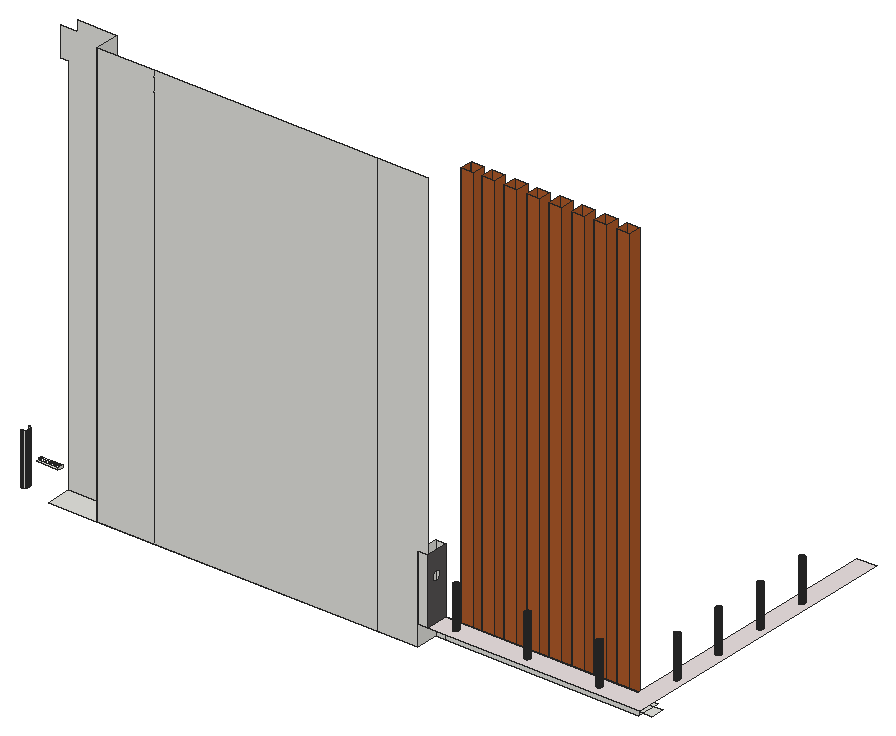
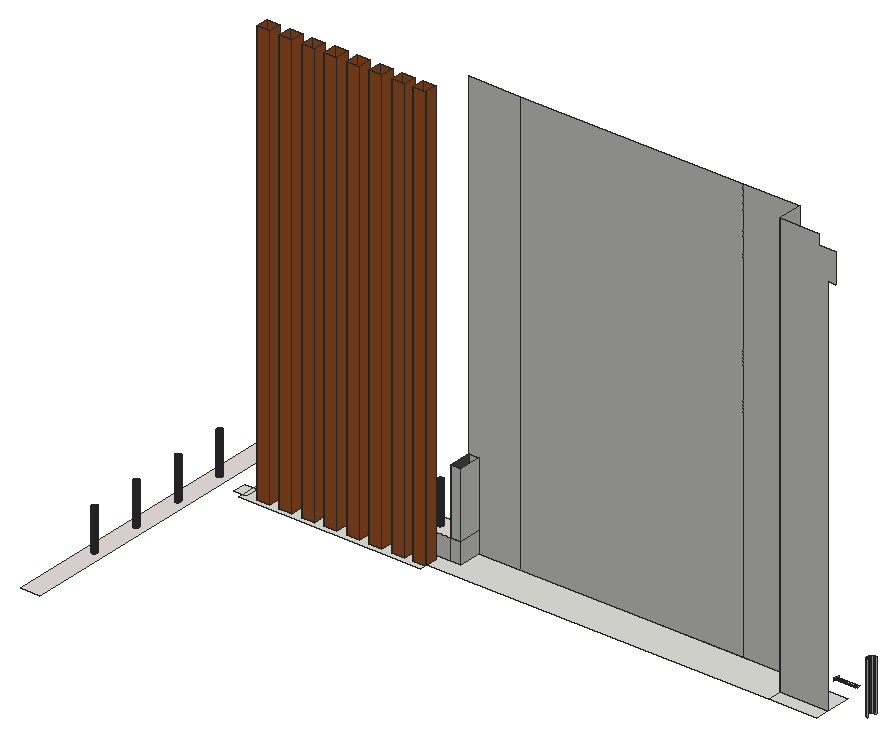
# SketchUp Ruby script. Lengths in inches.
U = 1.inch
M = Sketchup.active_model
def pt(a) = Geom::Point3d.new(a.map { |v| v * U })
def face(e, loops, mat)
  f = e.add_face(loops[0].map { |a| pt(a) })
  loops[1..].each { |l| e.add_face(l.map { |a| pt(a) }).erase! }
  f.material = f.back_material = mat if mat
  f
end
# faces: each face lists its corners as indices into pts; further lists are holes
def faces(e, pts, list, mat = nil) = list.each { |f| face(e, (f[0].is_a?(Array) ? f : [f]).map { |l| l.map { |i| pts[i] } }, mat) }
# xy, xz, yz: faces in a plane at the given z, y or x. An outline is a flat list of corners, or four numbers for a rectangle; further outlines are holes
def ring(l) = l.size == 4 ? [[l[0], l[1]], [l[2], l[1]], [l[2], l[3]], [l[0], l[3]]] : l.each_slice(2).to_a
def flat(e, list, mat, &to3) = list.each { |f| face(e, (f[0].is_a?(Array) ? f : [f]).map { |l| ring(l).map { |u, v| to3.(u, v) } }, mat) }
def xy(e, z, list, mat = nil) = flat(e, list, mat) { |x, y| [x, y, z] }
def xz(e, y, list, mat = nil) = flat(e, list, mat) { |x, z| [x, y, z] }
def yz(e, x, list, mat = nil) = flat(e, list, mat) { |y, z| [x, y, z] }
def lines(e, pts, list) = list.each { |a, b| e.add_line(pt(pts[a]), pt(pts[b])) }
# prism: a flat outline (further loops are holes) pulled along v
def prism(e, loops, v, mat = nil)
  f = face(e, loops, mat); d = Geom::Vector3d.new(v.map { |x| x * U })
  f.pushpull(f.normal.samedirection?(d) ? d.length : -d.length)
end
def box(e, o, s, mat = nil) = prism(e, [[o, [o[0] + s[0], o[1], o[2]], [o[0] + s[0], o[1] + s[1], o[2]], [o[0], o[1] + s[1], o[2]]]], [0, 0, s[2]], mat)
def at(x, y, z, deg = 0) = Geom::Transformation.translation(pt([x, y, z])) * Geom::Transformation.rotation(ORIGIN, Z_AXIS, deg.degrees)
def axes(o, x, y, z) = Geom::Transformation.new([*x, 0, *y, 0, *z, 0, *pt(o).to_a, 1])
def part(name) = M.definitions.add(name)
# library, detail: a bought-in or finely detailed component or shape, given as its bounding box
def library(name, o, s) = part(name).tap { |d| box(d.entities, o, s) }
def detail(e, o, s) = box(e.add_group.entities, o, s)
def put(e, d, t, mat = nil) = e.add_instance(d, t).tap { |i| i.material = mat if mat }
def group(e, t, mat = nil) = e.add_group.tap { |g| g.transformation = t; g.material = mat if mat }.entities
root = M.entities
M.materials.add("Generic\#2").color = [87, 84, 84]
M.materials.add("Generic\#6").color = [174, 89, 41]
M.materials.add("Generic\#9").color = [233, 223, 223]
M.materials.add("[Color M07]").color = [58, 58, 58]
xy(root,143.28,[[383.85,127.4375,394.85,133.125],[[394.85,127.4375,467.91,127.4375,467.91,132.5625,514.25,132.5625,514.25,133.85,513.34,133.85,513.34,136.78,514.25,136.78,514.25,138,472.76,138,472.76,136.78,475.69,136.78,475.69,133.85,472.76,133.85,472.76,136.1875,394.85,136.1875],[508.21,133.85,511.15,136.78],[503.09,133.85,506.03,136.78],[497.96,133.85,500.9,136.78],[492.84,133.85,495.78,136.78],[487.71,133.85,490.65,136.78],[482.59,133.85,485.53,136.78],[477.46,133.85,480.4,136.78]],[383.85,133.125,394.85,136.1875],[513.34,133.85,514.25,136.78],[514.25,133.85,516.28,136.78]])
xy(root,148.0625,[[467.91,127.4375,470.29,132.5625]])
xy(root,148.0625,[[[470.29,127.4375,518.6875,127.4375,518.6875,194.75,514.25,194.75,514.25,132.5625,470.29,132.5625],[516.54,175.625,516.38,175.65,516.23,175.71,516.1,175.81,516,175.9375,515.9375,176.09,515.92,176.25,515.9375,176.41,516,176.5625,516.1,176.69,516.23,176.79,516.38,176.85,516.54,176.875,516.7,176.85,516.86,176.79,516.98,176.69,517.08,176.5625,517.15,176.41,517.17,176.25,517.15,176.09,517.08,175.9375,516.98,175.81,516.86,175.71,516.7,175.65],[516.54,140,516.38,140.02,516.23,140.08,516.1,140.18,516,140.3125,515.9375,140.46,515.92,140.625,515.9375,140.79,516,140.9375,516.1,141.07,516.23,141.17,516.38,141.23,516.54,141.25,516.7,141.23,516.86,141.17,516.98,141.07,517.08,140.9375,517.15,140.79,517.17,140.625,517.15,140.46,517.08,140.3125,516.98,140.18,516.86,140.08,516.7,140.02],[516.54,151.875,516.38,151.9,516.23,151.96,516.1,152.06,516,152.1875,515.9375,152.34,515.92,152.5,515.9375,152.66,516,152.8125,516.1,152.94,516.23,153.04,516.38,153.1,516.54,153.125,516.7,153.1,516.86,153.04,516.98,152.94,517.08,152.8125,517.15,152.66,517.17,152.5,517.15,152.34,517.08,152.1875,516.98,152.06,516.86,151.96,516.7,151.9],[516.54,163.75,516.38,163.77,516.23,163.83,516.1,163.93,516,164.0625,515.9375,164.21,515.92,164.375,515.9375,164.54,516,164.6875,516.1,164.82,516.23,164.92,516.38,164.98,516.54,165,516.7,164.98,516.86,164.92,516.98,164.82,517.08,164.6875,517.15,164.54,517.17,164.375,517.15,164.21,517.08,164.0625,516.98,163.93,516.86,163.83,516.7,163.77],[490.99,129.43,490.83,129.45,490.68,129.51,490.55,129.61,490.45,129.74,490.39,129.89,490.37,130.05,490.39,130.21,490.45,130.36,490.55,130.49,490.68,130.59,490.83,130.66,490.99,130.68,491.15,130.66,491.3,130.59,491.43,130.49,491.53,130.36,491.59,130.21,491.62,130.05,491.59,129.89,491.53,129.74,491.43,129.61,491.3,129.51,491.15,129.45],[507.37,129.43,507.2,129.45,507.05,129.51,506.92,129.61,506.82,129.74,506.76,129.89,506.74,130.05,506.76,130.21,506.82,130.36,506.92,130.49,507.05,130.59,507.2,130.66,507.37,130.68,507.53,130.66,507.68,130.59,507.81,130.49,507.91,130.36,507.97,130.21,507.99,130.05,507.97,129.89,507.91,129.74,507.81,129.61,507.68,129.51,507.53,129.45],[474.62,129.43,474.45,129.45,474.3,129.51,474.17,129.61,474.07,129.74,474.01,129.89,473.99,130.05,474.01,130.21,474.07,130.36,474.17,130.49,474.3,130.59,474.45,130.66,474.62,130.68,474.78,130.66,474.93,130.59,475.06,130.49,475.16,130.36,475.22,130.21,475.24,130.05,475.22,129.89,475.16,129.74,475.06,129.61,474.93,129.51,474.78,129.45]]],"Generic\#9")
xy(root,148.75,[[378.85,130.19,383.85,130.82]])
xz(root,127.4375,[[394.85,143.28,407.84,240],[407.84,143.28,458.64,240],[458.64,143.28,458.64,240,470.29,240,470.29,162.875,467.91,162.875,467.91,143.28],[467.91,148.0625,470.29,162.875]])
xz(root,130.82,[[378.85,149.0625,383.85,149.1875],[378.85,149.0625,383.85,149.1875]])
xz(root,132.5625,[[467.91,143.28,470.29,148.0625],[470.29,143.28,514.25,148.0625],[467.91,148.0625,470.29,162.875]])
xz(root,133.125,[[383.85,143.28,383.85,231,381.97,231,381.97,237.6875,385.91,237.6875,385.91,240,394.85,240,394.85,143.28]])
xz(root,133.85,[[472.76,143.28,475.69,240],[477.46,143.28,480.4,240],[482.59,143.28,485.53,240],[487.71,143.28,490.65,240],[492.84,143.28,495.78,240],
  [497.96,143.28,500.9,240],[503.09,143.28,506.03,240],[508.21,143.28,511.15,240]],"Generic\#6")
xz(root,136.78,[[472.76,143.28,475.69,240],[477.46,143.28,480.4,240],[482.59,143.28,485.53,240],[487.71,143.28,490.65,240],[492.84,143.28,495.78,240],
  [497.96,143.28,500.9,240],[503.09,143.28,506.03,240],[508.21,143.28,511.15,240]],"Generic\#6")
yz(root,383.85,[[131.35,148.72,131.35,149.04,131.36,149.16,130.82,149.1875,130.82,149.0625,130.82,149.1875,130.19,149.1875,130.19,148.75,130.82,148.75]])
yz(root,394.85,[[127.4375,143.28,133.125,240]])
yz(root,467.91,[[127.4375,143.28,132.5625,148.0625],[127.4375,148.0625,132.5625,162.875]])
yz(root,470.29,[[[127.4375,148.0625,132.5625,162.875],[129.89,156.58,129.6,156.62,129.34,156.73,129.11,156.91,128.93,157.14,128.82,157.4,128.78,157.69,128.82,157.98,128.93,158.24,129.11,158.47,129.34,158.65,129.6,158.76,129.89,158.8,130.18,158.76,130.44,158.65,130.67,158.47,130.85,158.24,130.96,157.98,131,157.69,130.96,157.4,130.85,157.14,130.67,156.91,130.44,156.73,130.18,156.62]]],"Generic\#2")
yz(root,472.76,[[133.85,143.28,136.1875,240]],"Generic\#6")
yz(root,475.69,[[133.85,143.28,136.78,240]],"Generic\#6")
yz(root,477.46,[[133.85,143.28,136.78,240]],"Generic\#6")
yz(root,480.4,[[133.85,143.28,136.78,240]],"Generic\#6")
yz(root,482.59,[[133.85,143.28,136.78,240]],"Generic\#6")
yz(root,485.53,[[133.85,143.28,136.78,240]],"Generic\#6")
yz(root,487.71,[[133.85,143.28,136.78,240]],"Generic\#6")
yz(root,490.65,[[133.85,143.28,136.78,240]],"Generic\#6")
yz(root,492.84,[[133.85,143.28,136.78,240]],"Generic\#6")
yz(root,495.78,[[133.85,143.28,136.78,240]],"Generic\#6")
yz(root,497.96,[[133.85,143.28,136.78,240]],"Generic\#6")
yz(root,500.9,[[133.85,143.28,136.78,240]],"Generic\#6")
yz(root,503.09,[[133.85,143.28,136.78,240]],"Generic\#6")
yz(root,506.03,[[133.85,143.28,136.78,240]],"Generic\#6")
yz(root,508.21,[[133.85,143.28,136.78,240]],"Generic\#6")
yz(root,511.15,[[133.85,143.28,136.78,240]],"Generic\#6")
p = [[376.4,128.68,143.28],[376.66,128.64,143.28],[376.66,128.64,155.04],[376.4,128.68,155.04],[376.92,128.68,143.28],[376.92,128.68,155.04],
  [377.16,128.78,143.28],[377.16,128.78,155.04],[377.37,128.9375,143.28],[377.37,128.9375,155.04],[377.53,129.14,143.28],[377.53,129.14,155.04],
  [377.625,129.39,143.28],[377.625,129.39,155.04],[377.66,129.64,143.28],[377.66,129.64,155.04],[377.625,129.9,143.28],[377.625,129.9,155.04],
  [377.53,130.14,143.28],[377.53,130.14,155.04],[377.37,130.35,143.28],[377.37,130.35,155.04],[377.16,130.51,143.28],[377.16,130.51,155.04],
  [376.92,130.61,143.28],[376.92,130.61,155.04],[376.66,130.64,143.28],[376.66,130.64,155.04],[474.3,129.51,148.0625],[474.45,129.45,148.0625],
  [474.45,129.45,157.4],[474.3,129.51,157.4],[474.62,129.43,148.0625],[474.62,129.43,157.4],[474.78,129.45,148.0625],[474.78,129.45,157.4],
  [474.93,129.51,148.0625],[474.93,129.51,157.4],[490.68,129.51,148.0625],[490.83,129.45,148.0625],[490.83,129.45,157.4],[490.68,129.51,157.4],
  [490.99,129.43,148.0625],[490.99,129.43,157.4],[491.15,129.45,148.0625],[491.15,129.45,157.4],[491.3,129.51,148.0625],[491.3,129.51,157.4],
  [507.05,129.51,148.0625],[507.2,129.45,148.0625],[507.2,129.45,157.4],[507.05,129.51,157.4],[507.37,129.43,148.0625],[507.37,129.43,157.4],
  [507.53,129.45,148.0625],[507.53,129.45,157.4],[507.68,129.51,148.0625],[507.68,129.51,157.4],[474.17,129.61,148.0625],[474.17,129.61,157.4],
  [475.06,129.61,148.0625],[475.06,129.61,157.4],[490.55,129.61,148.0625],[490.55,129.61,157.4],[491.43,129.61,148.0625],[491.43,129.61,157.4],
  [506.92,129.61,148.0625],[506.92,129.61,157.4],[507.81,129.61,148.0625],[507.81,129.61,157.4],[474.07,129.74,148.0625],[474.07,129.74,157.4],
  [475.16,129.74,148.0625],[475.16,129.74,157.4],[490.45,129.74,148.0625],[490.45,129.74,157.4],[491.53,129.74,148.0625],[491.53,129.74,157.4],
  [506.82,129.74,148.0625],[506.82,129.74,157.4],[507.91,129.74,148.0625],[507.91,129.74,157.4],[474.01,129.89,148.0625],[474.01,129.89,157.4],
  [474.01,129.89,156.58],[475.22,129.89,148.0625],[475.22,129.89,156.58],[475.22,129.89,157.4],[490.39,129.89,148.0625],[490.39,129.89,157.4],
  [490.39,129.89,156.58],[491.59,129.89,148.0625],[491.59,129.89,156.58],[491.59,129.89,157.4],[506.76,129.89,148.0625],[506.76,129.89,157.4],
  [506.76,129.89,156.58],[507.97,129.89,148.0625],[507.97,129.89,156.58],[507.97,129.89,157.4],[473.99,130.05,148.0625],[473.99,130.05,157.4],
  [475.24,130.05,148.0625],[475.24,130.05,157.4],[490.37,130.05,148.0625],[490.37,130.05,157.4],[491.62,130.05,148.0625],[491.62,130.05,157.4],
  [506.74,130.05,148.0625],[506.74,130.05,157.4],[507.99,130.05,148.0625],[507.99,130.05,157.4],[474.01,130.21,148.0625],[474.01,130.21,157.4],
  [475.22,130.21,148.0625],[475.22,130.21,157.4],[490.39,130.21,148.0625],[490.39,130.21,157.4],[491.59,130.21,148.0625],[491.59,130.21,157.4],
  [506.76,130.21,148.0625],[506.76,130.21,157.4],[507.97,130.21,148.0625],[507.97,130.21,157.4],[474.07,130.36,148.0625],[474.07,130.36,157.4],
  [475.16,130.36,148.0625],[475.16,130.36,157.4],[490.45,130.36,148.0625],[490.45,130.36,157.4],[491.53,130.36,148.0625],[491.53,130.36,157.4],
  [506.82,130.36,148.0625],[506.82,130.36,157.4],[507.91,130.36,148.0625],[507.91,130.36,157.4],[474.17,130.49,148.0625],[474.17,130.49,157.4],
  [475.06,130.49,148.0625],[475.06,130.49,157.4],[490.55,130.49,148.0625],[490.55,130.49,157.4],[491.43,130.49,148.0625],[491.43,130.49,157.4],
  [506.92,130.49,148.0625],[506.92,130.49,157.4],[507.81,130.49,148.0625],[507.81,130.49,157.4],[474.3,130.59,148.0625],[474.3,130.59,157.4],
  [474.93,130.59,148.0625],[474.93,130.59,157.4],[490.68,130.59,148.0625],[490.68,130.59,157.4],[491.3,130.59,148.0625],[491.3,130.59,157.4],
  [507.05,130.59,148.0625],[507.05,130.59,157.4],[507.68,130.59,148.0625],[507.68,130.59,157.4],[474.45,130.66,148.0625],[474.45,130.66,157.4],
  [474.78,130.66,148.0625],[474.78,130.66,157.4],[490.83,130.66,148.0625],[490.83,130.66,157.4],[491.15,130.66,148.0625],[491.15,130.66,157.4],
  [507.2,130.66,148.0625],[507.2,130.66,157.4],[507.53,130.66,148.0625],[507.53,130.66,157.4],[474.62,130.68,148.0625],[474.62,130.68,157.4],
  [490.99,130.68,148.0625],[490.99,130.68,157.4],[507.37,130.68,148.0625],[507.37,130.68,157.4],[516.23,140.08,148.0625],[516.38,140.02,148.0625],
  [516.38,140.02,157.4],[516.23,140.08,157.4],[516.54,140,148.0625],[516.54,140,157.4],[516.7,140.02,148.0625],[516.7,140.02,156.58],
  [516.7,140.02,157.4],[516.86,140.08,148.0625],[516.86,140.08,157.4],[516.1,140.18,148.0625],[516.1,140.18,157.4],[516.98,140.18,148.0625],
  [516.98,140.18,157.4],[516,140.3125,148.0625],[516,140.3125,157.4],[517.08,140.3125,148.0625],[517.08,140.3125,157.4],[515.9375,140.46,148.0625],
  [515.9375,140.46,157.4],[517.15,140.46,148.0625],[517.15,140.46,157.4],[515.92,140.625,148.0625],[515.92,140.625,157.4],[517.17,140.625,148.0625],
  [517.17,140.625,157.4],[515.9375,140.79,148.0625],[515.9375,140.79,157.4],[517.15,140.79,148.0625],[517.15,140.79,157.4],[516,140.9375,148.0625],
  [516,140.9375,157.4],[517.08,140.9375,148.0625],[517.08,140.9375,157.4],[516.1,141.07,148.0625],[516.1,141.07,157.4],[516.98,141.07,148.0625],
  [516.98,141.07,157.4],[516.23,141.17,148.0625],[516.23,141.17,157.4],[516.86,141.17,148.0625],[516.86,141.17,157.4],[516.38,141.23,148.0625],
  [516.38,141.23,157.4],[516.54,141.25,148.0625],[516.54,141.25,157.4],[516.7,141.23,148.0625],[516.7,141.23,157.4],[516.7,141.23,156.58],
  [516.23,151.96,148.0625],[516.38,151.9,148.0625],[516.38,151.9,157.4],[516.23,151.96,157.4],[516.54,151.875,148.0625],[516.54,151.875,157.4],
  [516.7,151.9,148.0625],[516.7,151.9,156.58],[516.7,151.9,157.4],[516.86,151.96,148.0625],[516.86,151.96,157.4],[516.1,152.06,148.0625],
  [516.1,152.06,157.4],[516.98,152.06,148.0625],[516.98,152.06,157.4],[516,152.1875,148.0625],[516,152.1875,157.4],[517.08,152.1875,148.0625],
  [517.08,152.1875,157.4],[515.9375,152.34,148.0625],[515.9375,152.34,157.4],[517.15,152.34,148.0625],[517.15,152.34,157.4],[515.92,152.5,148.0625],
  [515.92,152.5,157.4],[517.17,152.5,148.0625],[517.17,152.5,157.4],[515.9375,152.66,148.0625],[515.9375,152.66,157.4],[517.15,152.66,148.0625],
  [517.15,152.66,157.4],[516,152.8125,148.0625],[516,152.8125,157.4],[517.08,152.8125,148.0625],[517.08,152.8125,157.4],[516.1,152.94,148.0625],
  [516.1,152.94,157.4],[516.98,152.94,148.0625],[516.98,152.94,157.4],[516.23,153.04,148.0625],[516.23,153.04,157.4],[516.86,153.04,148.0625],
  [516.86,153.04,157.4],[516.38,153.1,148.0625],[516.38,153.1,157.4],[516.7,153.1,148.0625],[516.7,153.1,156.58],[516.7,153.1,157.4],
  [516.54,153.125,148.0625],[516.54,153.125,157.4],[516.38,163.77,148.0625],[516.54,163.75,148.0625],[516.54,163.75,157.4],[516.38,163.77,157.4],
  [516.7,163.77,148.0625],[516.7,163.77,156.58],[516.7,163.77,157.4],[516.1,163.93,148.0625],[516.23,163.83,148.0625],[516.23,163.83,157.4],
  [516.1,163.93,157.4],[516.86,163.83,148.0625],[516.86,163.83,157.4],[516.98,163.93,148.0625],[516.98,163.93,157.4],[516,164.0625,148.0625],
  [516,164.0625,157.4],[517.08,164.0625,148.0625],[517.08,164.0625,157.4],[515.9375,164.21,148.0625],[515.9375,164.21,157.4],[517.15,164.21,148.0625],
  [517.15,164.21,157.4],[515.92,164.375,148.0625],[515.92,164.375,157.4],[517.17,164.375,148.0625],[517.17,164.375,157.4],[515.9375,164.54,148.0625],
  [515.9375,164.54,157.4],[517.15,164.54,148.0625],[517.15,164.54,157.4],[516,164.6875,148.0625],[516,164.6875,157.4],[517.08,164.6875,148.0625],
  [517.08,164.6875,157.4],[516.1,164.82,148.0625],[516.1,164.82,157.4],[516.98,164.82,148.0625],[516.98,164.82,157.4],[516.23,164.92,148.0625],
  [516.23,164.92,157.4],[516.86,164.92,148.0625],[516.86,164.92,157.4],[516.38,164.98,148.0625],[516.38,164.98,157.4],[516.7,164.98,148.0625],
  [516.7,164.98,156.58],[516.7,164.98,157.4],[516.54,165,148.0625],[516.54,165,157.4],[516.23,175.71,148.0625],[516.38,175.65,148.0625],
  [516.38,175.65,157.4],[516.23,175.71,157.4],[516.54,175.625,148.0625],[516.54,175.625,157.4],[516.7,175.65,148.0625],[516.7,175.65,156.58],
  [516.7,175.65,157.4],[516.86,175.71,148.0625],[516.86,175.71,157.4],[516.1,175.81,148.0625],[516.1,175.81,157.4],[516.98,175.81,148.0625],
  [516.98,175.81,157.4],[516,175.9375,148.0625],[516,175.9375,157.4],[517.08,175.9375,148.0625],[517.08,175.9375,157.4],[515.9375,176.09,148.0625],
  [515.9375,176.09,157.4],[517.15,176.09,148.0625],[517.15,176.09,157.4],[515.92,176.25,148.0625],[515.92,176.25,157.4],[517.17,176.25,148.0625],
  [517.17,176.25,157.4],[515.9375,176.41,148.0625],[515.9375,176.41,157.4],[517.15,176.41,148.0625],[517.15,176.41,157.4],[516,176.5625,148.0625],
  [516,176.5625,157.4],[517.08,176.5625,148.0625],[517.08,176.5625,157.4],[516.1,176.69,148.0625],[516.1,176.69,157.4],[516.98,176.69,148.0625],
  [516.98,176.69,157.4],[516.23,176.79,148.0625],[516.23,176.79,157.4],[516.86,176.79,148.0625],[516.86,176.79,157.4],[516.38,176.85,148.0625],
  [516.38,176.85,157.4],[516.7,176.85,148.0625],[516.7,176.85,156.58],[516.7,176.85,157.4],[516.54,176.875,148.0625],[516.54,176.875,157.4],
  [383.85,131.35,149.04],[378.85,131.35,149.04],[378.85,131.36,149.16],[383.85,131.36,149.16],[376.66,129.64,143.28],[376.66,129.64,155.47],
  [383.85,130.96,148.9],[378.85,130.96,148.9]]
faces(root,p,[[0,1,2,3],[1,4,5,2],[4,6,7,5],[6,8,9,7],[8,10,11,9],[10,12,13,11],[12,14,15,13],[14,16,17,15],
  [16,18,19,17],[18,20,21,19],[20,22,23,21],[22,24,25,23],[24,26,27,25],[378,379,380,381]])
faces(root,p,[[28,29,30,31],[29,32,33,30],[32,34,35,33],[34,36,37,35],[38,39,40,41],[39,42,43,40],[42,44,45,43],[44,46,47,45],
  [48,49,50,51],[49,52,53,50],[52,54,55,53],[54,56,57,55],[58,28,31,59],[36,60,61,37],[62,38,41,63],[46,64,65,47],
  [66,48,51,67],[56,68,69,57],[70,58,59,71],[60,72,73,61],[74,62,63,75],[64,76,77,65],[78,66,67,79],[68,80,81,69],
  [82,70,71,83,84],[72,85,86,87,73],[88,74,75,89,90],[76,91,92,93,77],[94,78,79,95,96],[80,97,98,99,81],[100,82,84,83,101],[85,102,103,87,86],
  [104,88,90,89,105],[91,106,107,93,92],[108,94,96,95,109],[97,110,111,99,98],[112,100,101,113],[102,114,115,103],[116,104,105,117],[106,118,119,107],
  [120,108,109,121],[110,122,123,111],[124,112,113,125],[114,126,127,115],[128,116,117,129],[118,130,131,119],[132,120,121,133],[122,134,135,123],
  [136,124,125,137],[126,138,139,127],[140,128,129,141],[130,142,143,131],[144,132,133,145],[134,146,147,135],[148,136,137,149],[138,150,151,139],
  [152,140,141,153],[142,154,155,143],[156,144,145,157],[146,158,159,147],[160,148,149,161],[150,162,163,151],[164,152,153,165],[154,166,167,155],
  [168,156,157,169],[158,170,171,159],[172,160,161,173],[162,172,173,163],[174,164,165,175],[166,174,175,167],[176,168,169,177],[170,176,177,171],
  [178,179,180,181],[179,182,183,180],[182,184,185,186,183],[184,187,188,186,185],[189,178,181,190],[187,191,192,188],[193,189,190,194],[191,195,196,192],
  [197,193,194,198],[195,199,200,196],[201,197,198,202],[199,203,204,200],[205,201,202,206],[203,207,208,204],[209,205,206,210],[207,211,212,208],
  [213,209,210,214],[211,215,216,212],[217,213,214,218],[215,219,220,216],[221,217,218,222],[223,221,222,224],[225,223,224,226,227],[219,225,227,226,220],
  [228,229,230,231],[229,232,233,230],[232,234,235,236,233],[234,237,238,236,235],[239,228,231,240],[237,241,242,238],[243,239,240,244],[241,245,246,242],
  [247,243,244,248],[245,249,250,246],[251,247,248,252],[249,253,254,250],[255,251,252,256],[253,257,258,254],[259,255,256,260],[257,261,262,258],
  [263,259,260,264],[261,265,266,262],[267,263,264,268],[265,269,270,266],[271,267,268,272],[269,273,274,275,270],[276,271,272,277],[273,276,277,275,274],
  [278,279,280,281],[279,282,283,284,280],[285,286,287,288],[286,278,281,287],[282,289,290,284,283],[289,291,292,290],[293,285,288,294],[291,295,296,292],
  [297,293,294,298],[295,299,300,296],[301,297,298,302],[299,303,304,300],[305,301,302,306],[303,307,308,304],[309,305,306,310],[307,311,312,308],
  [313,309,310,314],[311,315,316,312],[317,313,314,318],[315,319,320,316],[321,317,318,322],[319,323,324,325,320],[326,321,322,327],[323,326,327,325,324],
  [328,329,330,331],[329,332,333,330],[332,334,335,336,333],[334,337,338,336,335],[339,328,331,340],[337,341,342,338],[343,339,340,344],[341,345,346,342],
  [347,343,344,348],[345,349,350,346],[351,347,348,352],[349,353,354,350],[355,351,352,356],[353,357,358,354],[359,355,356,360],[357,361,362,358],
  [363,359,360,364],[361,365,366,362],[367,363,364,368],[365,369,370,366],[371,367,368,372],[369,373,374,375,370],[376,371,372,377],[373,376,377,375,374]],"[Color M07]")
lines(root,p,[[382,383],[384,385]])
